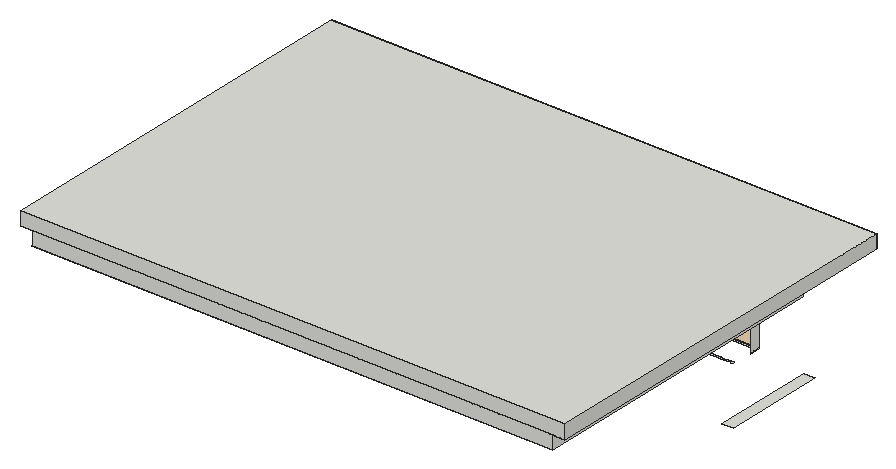
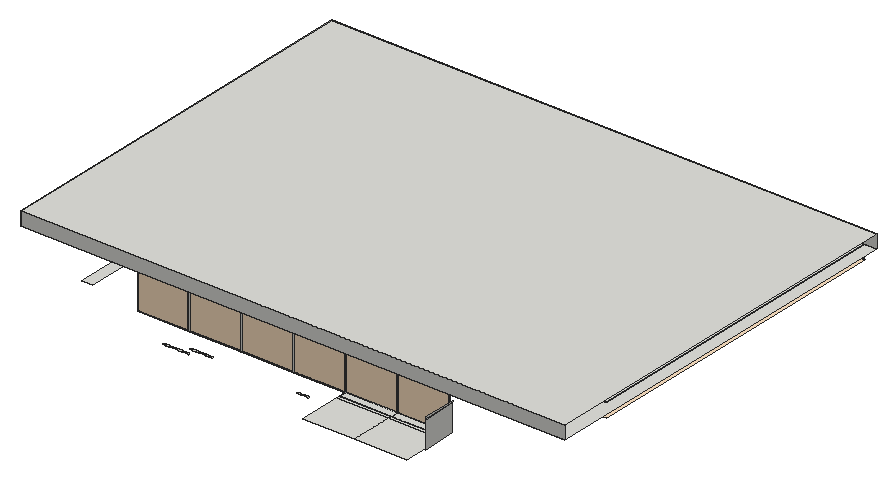
# SketchUp Ruby script. Lengths in inches.
U = 1.inch
M = Sketchup.active_model
def pt(a) = Geom::Point3d.new(a.map { |v| v * U })
def face(e, loops, mat)
  f = e.add_face(loops[0].map { |a| pt(a) })
  loops[1..].each { |l| e.add_face(l.map { |a| pt(a) }).erase! }
  f.material = f.back_material = mat if mat
  f
end
# faces: each face lists its corners as indices into pts; further lists are holes
def faces(e, pts, list, mat = nil) = list.each { |f| face(e, (f[0].is_a?(Array) ? f : [f]).map { |l| l.map { |i| pts[i] } }, mat) }
# xy, xz, yz: faces in a plane at the given z, y or x. An outline is a flat list of corners, or four numbers for a rectangle; further outlines are holes
def ring(l) = l.size == 4 ? [[l[0], l[1]], [l[2], l[1]], [l[2], l[3]], [l[0], l[3]]] : l.each_slice(2).to_a
def flat(e, list, mat, &to3) = list.each { |f| face(e, (f[0].is_a?(Array) ? f : [f]).map { |l| ring(l).map { |u, v| to3.(u, v) } }, mat) }
def xy(e, z, list, mat = nil) = flat(e, list, mat) { |x, y| [x, y, z] }
def xz(e, y, list, mat = nil) = flat(e, list, mat) { |x, z| [x, y, z] }
def yz(e, x, list, mat = nil) = flat(e, list, mat) { |y, z| [x, y, z] }
def lines(e, pts, list) = list.each { |a, b| e.add_line(pt(pts[a]), pt(pts[b])) }
# prism: a flat outline (further loops are holes) pulled along v
def prism(e, loops, v, mat = nil)
  f = face(e, loops, mat); d = Geom::Vector3d.new(v.map { |x| x * U })
  f.pushpull(f.normal.samedirection?(d) ? d.length : -d.length)
end
def box(e, o, s, mat = nil) = prism(e, [[o, [o[0] + s[0], o[1], o[2]], [o[0] + s[0], o[1] + s[1], o[2]], [o[0], o[1] + s[1], o[2]]]], [0, 0, s[2]], mat)
def at(x, y, z, deg = 0) = Geom::Transformation.translation(pt([x, y, z])) * Geom::Transformation.rotation(ORIGIN, Z_AXIS, deg.degrees)
def axes(o, x, y, z) = Geom::Transformation.new([*x, 0, *y, 0, *z, 0, *pt(o).to_a, 1])
def part(name) = M.definitions.add(name)
# library, detail: a bought-in or finely detailed component or shape, given as its bounding box
def library(name, o, s) = part(name).tap { |d| box(d.entities, o, s) }
def detail(e, o, s) = box(e.add_group.entities, o, s)
def put(e, d, t, mat = nil) = e.add_instance(d, t).tap { |i| i.material = mat if mat }
def group(e, t, mat = nil) = e.add_group.tap { |g| g.transformation = t; g.material = mat if mat }.entities
root = M.entities
M.materials.add("[0012_Bisque]").color = [255, 228, 196]
M.materials.add("[Color M08]").color = [30, 30, 30]
c1 = library("Group\#46",[0,0,0],[110.16,110.16,227.25])
xy(root,79.3125,[[188.65,140.48,188.84,140.5,189.01,140.57,189.16,140.6875,189.27,140.84,189.34,141.01,189.37,141.2,187.93,141.2,187.96,141.01,188.03,140.84,188.14,140.6875,188.29,140.57,188.46,140.5],[190.09,140.48,190.27,140.5,190.45,140.57,190.6,140.6875,190.71,140.84,190.78,141.01,190.81,141.2,189.37,141.2,189.39,141.01,189.46,140.84,189.58,140.6875,189.73,140.57,189.9,140.5],[191.52,140.48,191.71,140.5,191.88,140.57,192.03,140.6875,192.15,140.84,192.22,141.01,192.24,141.2,190.81,141.2,190.83,141.01,190.9,140.84,191.02,140.6875,191.17,140.57,191.34,140.5],[192.96,140.48,193.15,140.5,193.32,140.57,193.47,140.6875,193.58,140.84,193.66,141.01,193.68,141.2,192.24,141.2,192.27,141.01,192.34,140.84,192.45,140.6875,192.6,140.57,192.78,140.5],[194.4,140.48,194.59,140.5,194.76,140.57,194.91,140.6875,195.02,140.84,195.09,141.01,195.12,141.2,193.68,141.2,193.71,141.01,193.78,140.84,193.89,140.6875,194.04,140.57,194.21,140.5],
  [195.84,140.48,196.02,140.5,196.2,140.57,196.35,140.6875,196.46,140.84,196.53,141.01,196.56,141.2,195.12,141.2,195.14,141.01,195.21,140.84,195.33,140.6875,195.48,140.57,195.65,140.5],[197.27,140.48,197.46,140.5,197.63,140.57,197.78,140.6875,197.9,140.84,197.97,141.01,197.99,141.2,196.56,141.2,196.58,141.01,196.65,140.84,196.77,140.6875,196.92,140.57,197.09,140.5],[198.71,140.48,198.9,140.5,199.07,140.57,199.22,140.6875,199.33,140.84,199.35,140.87,199.35,141.2,197.99,141.2,198.02,141.01,198.09,140.84,198.2,140.6875,198.35,140.57,198.53,140.5]])
xy(root,80.75,[[136.42,140.54,136.58,140.54,136.65,140.55,136.73,140.57,136.8,140.59,136.94,140.66,137,140.7,137.07,140.75,137.12,140.8,137.22,140.92,137.26,140.98,137.29,141.05,137.3125,141.1,137.3,141.125,137.28,141.2,135.66,141.2,135.68,141.125,135.71,141.05,135.74,140.98,135.78,140.92,135.88,140.8,135.9375,140.75,136,140.7,136.0625,140.66,136.13,140.625,136.2,140.59,136.27,140.57,136.35,140.55],[138.05,140.54,138.2,140.54,138.28,140.55,138.35,140.57,138.43,140.59,138.57,140.66,138.63,140.7,138.75,140.8,138.8,140.86,138.88,140.98,138.92,141.05,138.9375,141.1,138.93,141.125,138.91,141.2,137.34,141.2,137.32,141.125,137.3125,141.1,137.33,141.05,137.37,140.98,137.45,140.86,137.51,140.8,137.5625,140.75,137.62,140.7,137.6875,140.66,137.75,140.625,137.83,140.59,137.97,140.55],[139.67,140.54,139.83,140.54,139.9,140.55,139.98,140.57,140.05,140.59,140.19,140.66,140.25,140.7,140.32,140.75,140.37,140.8,140.47,140.92,140.51,140.98,140.54,141.05,140.5625,141.1,140.55,141.125,140.53,141.2,138.97,141.2,138.95,141.125,138.9375,141.1,138.96,141.05,138.99,140.98,139.03,140.92,139.13,140.8,139.1875,140.75,139.25,140.7,139.3125,140.66,139.38,140.625,139.45,140.59,139.52,140.57,139.6,140.55]])
xy(root,81.5,[[178.38,140.48,178.57,140.5,178.74,140.57,178.89,140.6875,179,140.84,179.07,141.01,179.1,141.2,177.66,141.2,177.6875,141.01,177.76,140.84,177.87,140.6875,178.02,140.57,178.19,140.5],[179.82,140.48,180,140.5,180.18,140.57,180.33,140.6875,180.44,140.84,180.51,141.01,180.54,141.2,179.1,141.2,179.125,141.01,179.19,140.84,179.31,140.6875,179.46,140.57,179.63,140.5],[181.25,140.48,181.44,140.5,181.61,140.57,181.76,140.6875,181.88,140.84,181.95,141.01,181.97,141.2,180.54,141.2,180.5625,141.01,180.63,140.84,180.75,140.6875,180.9,140.57,181.07,140.5],[182.69,140.48,182.88,140.5,183.05,140.57,183.2,140.6875,183.31,140.84,183.39,141.01,183.41,141.2,181.97,141.2,182,141.01,182.07,140.84,182.18,140.6875,182.33,140.57,182.51,140.5],[184.13,140.48,184.32,140.5,184.49,140.57,184.64,140.6875,184.75,140.84,184.82,141.01,184.85,141.2,183.41,141.2,183.4375,141.01,183.51,140.84,183.62,140.6875,183.77,140.57,183.94,140.5],
  [185.57,140.48,185.75,140.5,185.93,140.57,186.08,140.6875,186.19,140.84,186.26,141.01,186.29,141.2,184.85,141.2,184.875,141.01,184.94,140.84,185.06,140.6875,185.21,140.57,185.38,140.5],[186.96,140.52,187.13,140.55,187.29,140.61,187.43,140.72,187.54,140.86,187.61,141.02,187.63,141.2,186.29,141.2,186.31,141.02,186.375,140.86,186.48,140.72,186.62,140.61,186.78,140.55]])
xy(root,88.4375,[[119.1875,139.88,142,141.2],[142.3,139.88,164.82,141.2],[164.82,139.88,187.63,141.2],[187.93,139.88,210.45,141.2],[73.56,141.2,96.375,144.68],
  [96.375,141.2,119.1875,144.68],[96.375,144.68,96.75,144.86]])
xy(root,88.6875,[[233.26,92.18,238.375,136.82],[73.56,141.2,73.86,141.5],[73.86,141.2,96.375,141.2,96.375,144.68,73.56,144.68,73.56,141.5,73.86,141.5],[96.375,141.2,96.67,141.5],[96.67,141.2,119.1875,141.2,119.1875,144.68,96.375,144.68,96.375,141.5,96.67,141.5],
  [119.1875,141.2,119.49,141.5],[142,141.2,142.3,141.5],[164.82,141.2,165.12,141.5],[187.63,141.2,187.93,141.5],[73.56,144.68,96.375,146.09],
  [96.375,144.68,119.1875,146.09],[73.56,146.09,96.375,164.88],[96.375,146.09,119.1875,164.88]])
xy(root,118.75,[[14.13,9.32,14.13,113.7,15.9375,113.7,15.9375,11.12,221.84,11.12,221.84,40.08,223.64,40.08,223.64,9.32],[221.84,70.84,223.64,105.76],[84.16,130.07,112.09,131.88],[169.24,130.07,210.41,131.88]])
xy(root,118.75,[[[4.82,0,4.82,141.2,27.63,141.2,27.63,141.5,27.93,141.5,27.93,141.2,50.14,141.2,50.14,141.5,50.44,141.5,50.44,141.2,73.26,141.2,73.26,141.5,73.56,141.5,73.56,141.2,96.07,141.2,96.07,141.5,96.375,141.5,96.375,141.2,118.89,141.2,118.89,141.5,119.1875,141.5,119.1875,141.2,141.7,141.2,141.7,141.5,142,141.5,142,141.2,164.52,141.2,164.52,141.5,164.82,141.5,164.82,141.2,187.33,141.2,187.33,141.5,187.63,141.5,187.63,141.2,210.15,141.2,210.15,136.82,232.96,136.82,232.96,0],[14.13,9.32,223.64,131.88]],[[15.9375,11.12,221.84,130.07],[27.94,23.13,209.83,23.13,209.83,113.69,210.21,118.07,27.94,118.07]]],"[0012_Bisque]")
xy(root,118.75,[[221.84,40.08,223.64,70.84],[221.84,105.76,221.84,130.07,210.41,130.07,210.41,131.88,223.64,131.88,223.64,105.76],[112.09,130.07,169.24,131.88]],"[Color M08]")
xy(root,122.5625,[[27.94,23.13,27.94,118.07,210.21,118.07,209.83,113.69,209.83,23.13]],"[0012_Bisque]")
xy(root,124.6875,[[0,0,0,170.3125,238.375,170.3125,238.375,0,233.26,0,233.26,136.82,210.45,136.82,210.45,141.2,187.93,141.2,187.93,141.5,187.33,141.5,187.33,141.2,165.12,141.2,165.12,141.5,164.52,141.5,164.52,141.2,142.3,141.2,142.3,141.5,141.7,141.5,141.7,141.2,119.49,141.2,119.49,141.5,118.89,141.5,118.89,141.2,96.67,141.2,96.67,141.5,96.07,141.5,96.07,141.2,73.86,141.2,73.86,141.5,73.26,141.5,73.26,141.2,50.74,141.2,50.74,141.5,50.14,141.5,50.14,141.2,28.23,141.2,28.23,141.5,27.63,141.5,27.63,141.2,4.82,141.2,4.82,0],[5.62,0,232.96,0,232.96,136.82,210.15,136.82,210.15,141.2,5.62,141.2],[232.96,0,233.26,136.82],[210.15,136.82,210.45,141.2],[73.26,141.2,73.56,141.5],
  [73.56,141.2,73.86,141.5],[96.07,141.2,96.375,141.5],[96.375,141.2,96.67,141.5],[118.89,141.2,119.1875,141.5],[119.1875,141.2,119.49,141.5],
  [141.7,141.2,142,141.5],[142,141.2,142.3,141.5],[164.52,141.2,164.82,141.5],[164.82,141.2,165.12,141.5],[187.33,141.2,187.63,141.5],
  [187.63,141.2,187.93,141.5]])
xy(root,130.6875,[[0,0,238.375,170.3125]])
xz(root,0,[[5.62,118.75,232.96,124.6875],[0,124.6875,238.375,130.6875]])
xz(root,23.13,[[27.94,118.75,209.83,122.5625]])
xz(root,118.07,[[27.94,118.75,210.21,122.5625]],"[0012_Bisque]")
xz(root,136.82,[[210.15,118.75,210.45,124.6875],[210.45,118.75,232.96,124.6875]])
xz(root,141.2,[[73.56,88.4375,96.375,88.6875],[96.375,88.4375,119.1875,88.6875],[119.1875,88.4375,142,88.6875],[142,88.4375,164.82,88.6875],[164.82,88.4375,187.63,88.6875],
  [187.63,88.4375,210.45,88.6875],[73.56,118.75,73.86,124.6875],[73.86,118.75,96.07,124.6875],[96.375,118.75,96.67,124.6875],[96.67,118.75,118.89,124.6875],
  [119.1875,118.75,119.49,124.6875],[119.49,118.75,141.7,124.6875],[142,118.75,142.3,124.6875],[142.3,118.75,164.52,124.6875],[164.82,118.75,165.12,124.6875],
  [165.12,118.75,187.33,124.6875],[187.63,118.75,187.93,124.6875],[187.93,118.75,210.15,124.6875]])
xz(root,141.2,[[73.86,88.6875,96.375,88.6875,96.375,124.6875,96.07,124.6875,96.07,118.75,73.86,118.75],[96.67,88.6875,119.1875,88.6875,119.1875,124.6875,118.89,124.6875,118.89,118.75,96.67,118.75],[119.49,88.6875,142,88.6875,142,124.6875,141.7,124.6875,141.7,118.75,119.49,118.75],[142.3,88.6875,164.82,88.6875,164.82,124.6875,164.52,124.6875,164.52,118.75,142.3,118.75],[165.12,88.6875,187.63,88.6875,187.63,124.6875,187.33,124.6875,187.33,118.75,165.12,118.75],
  [187.93,88.6875,210.45,88.6875,210.45,124.6875,210.15,124.6875,210.15,118.75,187.93,118.75]],"[0012_Bisque]")
xz(root,141.5,[[73.56,88.6875,73.86,124.6875],[96.375,88.6875,96.67,124.6875],[119.1875,88.6875,119.49,124.6875],[142,88.6875,142.3,124.6875],[164.82,88.6875,165.12,124.6875],
  [187.63,88.6875,187.93,124.6875],[73.26,118.75,73.56,124.6875],[96.07,118.75,96.375,124.6875],[118.89,118.75,119.1875,124.6875],[141.7,118.75,142,124.6875],
  [164.52,118.75,164.82,124.6875],[187.33,118.75,187.63,124.6875]])
xz(root,144.68,[[73.56,88.4375,96.375,88.6875],[96.375,88.4375,119.1875,88.6875]])
xz(root,170.3125,[[0,124.6875,238.375,130.6875]])
yz(root,72.61,[[141.2,88.95,155.95,100.6875]])
yz(root,73.26,[[141.2,118.75,141.5,124.6875]])
yz(root,73.56,[[141.2,88.4375,144.68,88.6875],[141.2,88.6875,141.5,100.6875],[141.2,100.6875,141.5,118.75],[141.2,118.75,141.5,124.6875]])
yz(root,73.86,[[141.2,88.6875,141.5,100.6875],[141.2,100.6875,141.5,124.6875]])
yz(root,96.07,[[141.2,118.75,141.5,124.6875]])
yz(root,96.375,[[141.2,88.4375,144.68,88.6875],[141.2,88.6875,141.5,118.75],[141.2,118.75,141.5,124.6875]])
yz(root,96.67,[[141.2,88.6875,141.5,124.6875]])
yz(root,118.89,[[141.2,118.75,141.5,124.6875]])
yz(root,119.1875,[[141.2,88.4375,144.68,88.6875],[141.2,88.6875,141.5,118.75],[141.2,118.75,141.5,124.6875]])
yz(root,119.49,[[141.2,88.6875,141.5,124.6875]])
yz(root,141.7,[[141.2,118.75,141.5,124.6875]])
yz(root,142,[[141.2,88.6875,141.5,118.75],[141.2,118.75,141.5,124.6875]])
yz(root,142.3,[[141.2,88.6875,141.5,124.6875]])
yz(root,164.52,[[141.2,118.75,141.5,124.6875]])
yz(root,164.82,[[141.2,88.6875,141.5,118.75],[141.2,118.75,141.5,124.6875]])
yz(root,165.12,[[141.2,88.6875,141.5,124.6875]])
yz(root,187.33,[[141.2,118.75,141.5,124.6875]])
yz(root,187.63,[[141.2,88.6875,141.5,118.75],[141.2,118.75,141.5,124.6875]])
yz(root,187.93,[[141.2,88.6875,141.5,124.6875]])
yz(root,209.83,[[23.13,118.75,113.69,122.5625]],"[0012_Bisque]")
yz(root,210.15,[[136.82,118.75,141.2,124.6875]])
yz(root,210.45,[[136.82,88.4375,141.2,88.6875],[136.82,88.6875,141.2,124.6875]])
yz(root,232.96,[[0,118.75,136.82,124.6875]])
yz(root,238.375,[[0,124.6875,170.3125,130.6875]])
p = [[72.61,141.2,100.6875],[72.59,141.2,101.23],[72.59,155.95,101.23],[72.61,155.95,100.6875],[72.55,141.2,101.78],[72.55,155.95,101.78],
  [210.21,118.07,118.75],[209.83,113.69,118.75],[209.83,113.69,122.5625],[210.21,118.07,122.5625]]
faces(root,p,[[0,1,2,3],[1,4,5,2],[6,7,8,9]])
put(root,c1,axes([115.63,109.31,85.03],[0.14,0,0],[0,0.14,0],[0,0,0.14]))
put(root,c1,axes([175.07,109.31,85.03],[0.14,0,0],[0,0.14,0],[0,0,0.14]))
